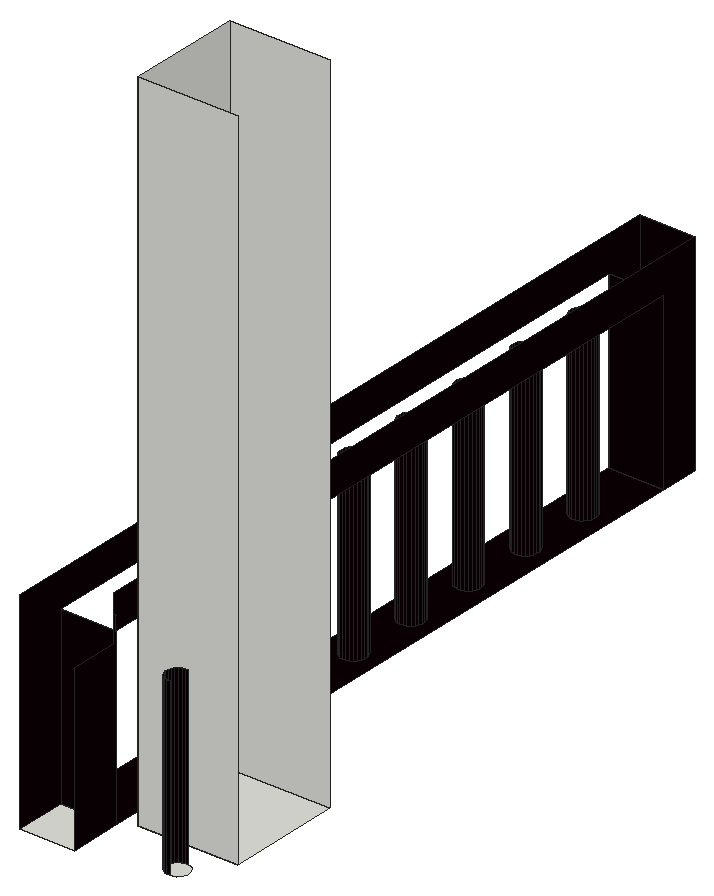
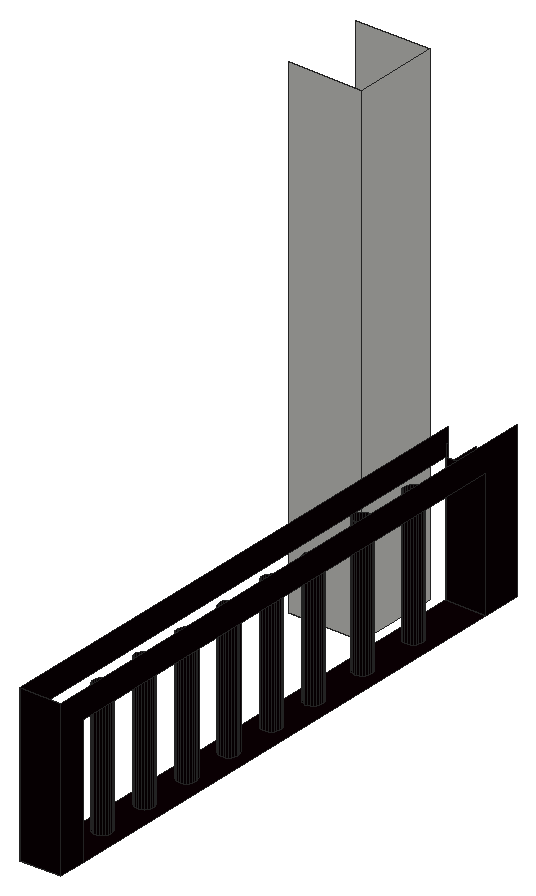
# SketchUp Ruby script. Lengths in inches.
U = 1.inch
M = Sketchup.active_model
def pt(a) = Geom::Point3d.new(a.map { |v| v * U })
def face(e, loops, mat)
  f = e.add_face(loops[0].map { |a| pt(a) })
  loops[1..].each { |l| e.add_face(l.map { |a| pt(a) }).erase! }
  f.material = f.back_material = mat if mat
  f
end
# faces: each face lists its corners as indices into pts; further lists are holes
def faces(e, pts, list, mat = nil) = list.each { |f| face(e, (f[0].is_a?(Array) ? f : [f]).map { |l| l.map { |i| pts[i] } }, mat) }
# xy, xz, yz: faces in a plane at the given z, y or x. An outline is a flat list of corners, or four numbers for a rectangle; further outlines are holes
def ring(l) = l.size == 4 ? [[l[0], l[1]], [l[2], l[1]], [l[2], l[3]], [l[0], l[3]]] : l.each_slice(2).to_a
def flat(e, list, mat, &to3) = list.each { |f| face(e, (f[0].is_a?(Array) ? f : [f]).map { |l| ring(l).map { |u, v| to3.(u, v) } }, mat) }
def xy(e, z, list, mat = nil) = flat(e, list, mat) { |x, y| [x, y, z] }
def xz(e, y, list, mat = nil) = flat(e, list, mat) { |x, z| [x, y, z] }
def yz(e, x, list, mat = nil) = flat(e, list, mat) { |y, z| [x, y, z] }
def lines(e, pts, list) = list.each { |a, b| e.add_line(pt(pts[a]), pt(pts[b])) }
# prism: a flat outline (further loops are holes) pulled along v
def prism(e, loops, v, mat = nil)
  f = face(e, loops, mat); d = Geom::Vector3d.new(v.map { |x| x * U })
  f.pushpull(f.normal.samedirection?(d) ? d.length : -d.length)
end
def box(e, o, s, mat = nil) = prism(e, [[o, [o[0] + s[0], o[1], o[2]], [o[0] + s[0], o[1] + s[1], o[2]], [o[0], o[1] + s[1], o[2]]]], [0, 0, s[2]], mat)
def at(x, y, z, deg = 0) = Geom::Transformation.translation(pt([x, y, z])) * Geom::Transformation.rotation(ORIGIN, Z_AXIS, deg.degrees)
def axes(o, x, y, z) = Geom::Transformation.new([*x, 0, *y, 0, *z, 0, *pt(o).to_a, 1])
def part(name) = M.definitions.add(name)
# library, detail: a bought-in or finely detailed component or shape, given as its bounding box
def library(name, o, s) = part(name).tap { |d| box(d.entities, o, s) }
def detail(e, o, s) = box(e.add_group.entities, o, s)
def put(e, d, t, mat = nil) = e.add_instance(d, t).tap { |i| i.material = mat if mat }
def group(e, t, mat = nil) = e.add_group.tap { |g| g.transformation = t; g.material = mat if mat }.entities
root = M.entities
M.materials.add("[Metal Seamed]").color = [11, 0, 4]
xy(root,148.4375,[[12.3125,62.41,21.75,71.24],[35.91,65.07,35.4,65.08,34.92,65.22,34.48,65.48,34.13,65.84,33.89,66.29,33.76,66.78,33.77,67.28,33.91,67.77,34.17,68.2,34.53,68.55,34.98,68.8,35.47,68.92,35.97,68.91,36.46,68.78,36.89,68.52,37.25,68.15,37.49,67.71,37.61,67.22,37.61,66.71,37.47,66.23,37.21,65.79,36.84,65.44,36.4,65.2],[24.07,73.08,41.19,92.83],[17.07,84.28,16.52,84.4,16.03,84.65,15.62,85.02,15.32,85.49,15.15,86.02,15.125,86.57,15.24,87.12,15.5,87.61,15.87,88.02,16.34,88.32,16.87,88.49,17.42,88.51,17.96,88.4,18.45,88.14,18.87,87.77,19.17,87.3,19.33,86.77,19.36,86.22,19.24,85.68,18.99,85.19,18.62,84.77,18.15,84.47,17.62,84.31],[17.07,99.09,16.52,99.21,16.03,99.46,15.62,99.84,15.32,100.3,15.15,100.83,15.125,101.39,15.24,101.93,15.5,102.42,15.87,102.83,16.34,103.13,16.87,103.3,17.42,103.33,17.96,103.21,18.45,102.96,18.87,102.58,19.17,102.12,19.33,101.59,19.36,101.03,19.24,100.49,18.99,100,18.62,99.59,18.15,99.29,17.62,99.12],
  [17.07,113.4,16.52,113.52,16.03,113.78,15.62,114.15,15.32,114.62,15.15,115.14,15.125,115.7,15.24,116.24,15.5,116.73,15.87,117.14,16.34,117.44,16.87,117.61,17.42,117.64,17.96,117.52,18.45,117.27,18.87,116.89,19.17,116.43,19.33,115.9,19.36,115.35,19.24,114.8,18.99,114.31,18.62,113.9,18.15,113.6,17.62,113.43],[17.07,125.72,16.52,125.83,16.03,126.09,15.62,126.46,15.32,126.93,15.15,127.46,15.125,128.01,15.24,128.55,15.5,129.05,15.87,129.46,16.34,129.76,16.87,129.93,17.42,129.95,17.96,129.83,18.45,129.58,18.87,129.21,19.17,128.74,19.33,128.21,19.36,127.66,19.24,127.12,18.99,126.62,18.62,126.21,18.15,125.91,17.62,125.74],[17.07,138.03,16.52,138.15,16.03,138.4,15.62,138.77,15.32,139.24,15.15,139.77,15.125,140.32,15.24,140.87,15.5,141.36,15.87,141.77,16.34,142.07,16.87,142.24,17.42,142.26,17.96,142.15,18.45,141.89,18.87,141.52,19.17,141.05,19.33,140.52,19.36,139.97,19.24,139.43,18.99,138.94,18.62,138.52,18.15,138.22,17.62,138.06],[17.07,150.34,16.52,150.46,16.03,150.71,15.62,151.09,15.32,151.55,15.15,152.08,15.125,152.64,15.24,153.18,15.5,153.67,15.87,154.08,16.34,154.38,16.87,154.55,17.42,154.58,17.96,154.46,18.45,154.21,18.87,153.83,19.17,153.37,19.33,152.84,19.36,152.28,19.24,151.74,18.99,151.25,18.62,150.84,18.15,150.54,17.62,150.37],[17.07,162.65,16.52,162.77,16.03,163.03,15.62,163.4,15.32,163.87,15.15,164.39,15.125,164.95,15.24,165.49,15.5,165.98,15.87,166.39,16.34,166.69,16.87,166.86,17.42,166.89,17.96,166.77,18.45,166.52,18.87,166.14,19.17,165.68,19.33,165.15,19.36,164.6,19.24,164.05,18.99,163.56,18.62,163.15,18.15,162.85,17.62,162.68],
  [17.07,174.97,16.52,175.08,16.03,175.34,15.62,175.71,15.32,176.18,15.15,176.71,15.125,177.26,15.24,177.8,15.5,178.3,15.87,178.71,16.34,179.01,16.87,179.18,17.42,179.2,17.96,179.08,18.45,178.83,18.87,178.46,19.17,177.99,19.33,177.46,19.36,176.91,19.24,176.37,18.99,175.87,18.62,175.46,18.15,175.16,17.62,174.99],[12.3125,188.85,21.75,195.41]])
xy(root,148.4375,[[[12.3125,71.24,21.75,188.85],[17.07,162.65,16.52,162.77,16.03,163.03,15.62,163.4,15.32,163.87,15.15,164.39,15.125,164.95,15.24,165.49,15.5,165.98,15.87,166.39,16.34,166.69,16.87,166.86,17.42,166.89,17.96,166.77,18.45,166.52,18.87,166.14,19.17,165.68,19.33,165.15,19.36,164.6,19.24,164.05,18.99,163.56,18.62,163.15,18.15,162.85,17.62,162.68],[17.07,150.34,16.52,150.46,16.03,150.71,15.62,151.09,15.32,151.55,15.15,152.08,15.125,152.64,15.24,153.18,15.5,153.67,15.87,154.08,16.34,154.38,16.87,154.55,17.42,154.58,17.96,154.46,18.45,154.21,18.87,153.83,19.17,153.37,19.33,152.84,19.36,152.28,19.24,151.74,18.99,151.25,18.62,150.84,18.15,150.54,17.62,150.37],[17.07,138.03,16.52,138.15,16.03,138.4,15.62,138.77,15.32,139.24,15.15,139.77,15.125,140.32,15.24,140.87,15.5,141.36,15.87,141.77,16.34,142.07,16.87,142.24,17.42,142.26,17.96,142.15,18.45,141.89,18.87,141.52,19.17,141.05,19.33,140.52,19.36,139.97,19.24,139.43,18.99,138.94,18.62,138.52,18.15,138.22,17.62,138.06],[17.07,125.72,16.52,125.83,16.03,126.09,15.62,126.46,15.32,126.93,15.15,127.46,15.125,128.01,15.24,128.55,15.5,129.05,15.87,129.46,16.34,129.76,16.87,129.93,17.42,129.95,17.96,129.83,18.45,129.58,18.87,129.21,19.17,128.74,19.33,128.21,19.36,127.66,19.24,127.12,18.99,126.62,18.62,126.21,18.15,125.91,17.62,125.74],[17.07,113.4,16.52,113.52,16.03,113.78,15.62,114.15,15.32,114.62,15.15,115.14,15.125,115.7,15.24,116.24,15.5,116.73,15.87,117.14,16.34,117.44,16.87,117.61,17.42,117.64,17.96,117.52,18.45,117.27,18.87,116.89,19.17,116.43,19.33,115.9,19.36,115.35,19.24,114.8,18.99,114.31,18.62,113.9,18.15,113.6,17.62,113.43],[17.07,99.09,16.52,99.21,16.03,99.46,15.62,99.84,15.32,100.3,15.15,100.83,15.125,101.39,15.24,101.93,15.5,102.42,15.87,102.83,16.34,103.13,16.87,103.3,17.42,103.33,17.96,103.21,18.45,102.96,18.87,102.58,19.17,102.12,19.33,101.59,19.36,101.03,19.24,100.49,18.99,100,18.62,99.59,18.15,99.29,17.62,99.12],[17.07,84.28,16.52,84.4,16.03,84.65,15.62,85.02,15.32,85.49,15.15,86.02,15.125,86.57,15.24,87.12,15.5,87.61,15.87,88.02,16.34,88.32,16.87,88.49,17.42,88.51,17.96,88.4,18.45,88.14,18.87,87.77,19.17,87.3,19.33,86.77,19.36,86.22,19.24,85.68,18.99,85.19,18.62,84.77,18.15,84.47,17.62,84.31],[17.07,174.97,16.52,175.08,16.03,175.34,15.62,175.71,15.32,176.18,15.15,176.71,15.125,177.26,15.24,177.8,15.5,178.3,15.87,178.71,16.34,179.01,16.87,179.18,17.42,179.2,17.96,179.08,18.45,178.83,18.87,178.46,19.17,177.99,19.33,177.46,19.36,176.91,19.24,176.37,18.99,175.87,18.62,175.46,18.15,175.16,17.62,174.99]]],"[Metal Seamed]")
xz(root,71.24,[[12.3125,148.4375,21.75,178.35]],"[Metal Seamed]")
xz(root,73.08,[[24.07,148.4375,41.19,263.5625]])
xz(root,92.83,[[24.07,148.4375,41.19,263.5625]])
xz(root,188.85,[[12.3125,148.4375,21.75,178.35]],"[Metal Seamed]")
xz(root,195.41,[[12.3125,148.4375,21.75,184.4375]],"[Metal Seamed]")
yz(root,12.3125,[[62.41,148.4375,62.41,184.4375,195.41,184.4375,195.41,148.4375,188.85,148.4375,188.85,178.35,71.24,178.35,71.24,148.4375]],"[Metal Seamed]")
yz(root,21.75,[[62.41,148.4375,71.24,148.4375,71.24,181.04,70.73,181.04,70.73,176.54,62.41,176.54],[188.85,148.4375,195.41,148.4375,195.41,184.4375,70.73,184.4375,70.73,181.04,71.24,181.04,71.24,178.35,188.85,178.35]],"[Metal Seamed]")
yz(root,24.07,[[73.08,148.4375,92.83,263.5625]])
p = [[34.92,65.22,148.4375],[35.4,65.08,148.4375],[35.4,65.08,178.3125],[34.92,65.22,178.3125],[35.91,65.07,148.4375],[35.91,65.07,178.3125],
  [34.48,65.48,148.4375],[34.48,65.48,178.3125],[34.13,65.84,148.4375],[34.13,65.84,178.3125],[33.89,66.29,148.4375],[33.89,66.29,178.3125],
  [33.76,66.78,148.4375],[33.76,66.78,178.3125],[33.77,67.28,148.4375],[33.77,67.28,178.3125],[33.91,67.77,148.4375],[33.91,67.77,178.3125],
  [34.17,68.2,148.4375],[34.17,68.2,178.3125],[34.53,68.55,148.4375],[34.53,68.55,178.3125],[34.98,68.8,148.4375],[34.98,68.8,178.3125],
  [35.47,68.92,148.4375],[35.47,68.92,178.3125],[35.97,68.91,148.4375],[35.97,68.91,178.3125],[16.52,84.4,148.4375],[17.07,84.28,148.4375],
  [17.07,84.28,179.5625],[16.52,84.4,179.5625],[17.62,84.31,148.4375],[17.62,84.31,179.5625],[18.15,84.47,148.4375],[18.15,84.47,179.5625],
  [16.03,84.65,148.4375],[16.03,84.65,179.5625],[18.62,84.77,148.4375],[18.62,84.77,179.5625],[15.62,85.02,148.4375],[15.62,85.02,179.5625],
  [18.99,85.19,148.4375],[18.99,85.19,179.5625],[15.32,85.49,148.4375],[15.32,85.49,179.5625],[19.24,85.68,148.4375],[19.24,85.68,179.5625],
  [15.15,86.02,148.4375],[15.15,86.02,179.5625],[19.36,86.22,148.4375],[19.36,86.22,179.5625],[15.125,86.57,148.4375],[15.125,86.57,179.5625],
  [19.33,86.77,148.4375],[19.33,86.77,179.5625],[15.24,87.12,148.4375],[15.24,87.12,179.5625],[19.17,87.3,148.4375],[19.17,87.3,179.5625],
  [15.5,87.61,148.4375],[15.5,87.61,179.5625],[18.87,87.77,148.4375],[18.87,87.77,179.5625],[15.87,88.02,148.4375],[15.87,88.02,179.5625],
  [18.45,88.14,148.4375],[18.45,88.14,179.5625],[16.34,88.32,148.4375],[16.34,88.32,179.5625],[17.96,88.4,148.4375],[17.96,88.4,179.5625],
  [16.87,88.49,148.4375],[16.87,88.49,179.5625],[17.42,88.51,148.4375],[17.42,88.51,179.5625],[16.52,99.21,148.4375],[17.07,99.09,148.4375],
  [17.07,99.09,180.25],[16.52,99.21,180.25],[17.62,99.12,148.4375],[17.62,99.12,180.25],[18.15,99.29,148.4375],[18.15,99.29,180.25],
  [16.03,99.46,148.4375],[16.03,99.46,180.25],[18.62,99.59,148.4375],[18.62,99.59,180.25],[15.62,99.84,148.4375],[15.62,99.84,180.25],
  [18.99,100,148.4375],[18.99,100,180.25],[15.32,100.3,148.4375],[15.32,100.3,180.25],[19.24,100.49,148.4375],[19.24,100.49,180.25],
  [15.15,100.83,148.4375],[15.15,100.83,180.25],[19.36,101.03,148.4375],[19.36,101.03,180.25],[15.125,101.39,148.4375],[15.125,101.39,180.25],
  [19.33,101.59,148.4375],[19.33,101.59,180.25],[15.24,101.93,148.4375],[15.24,101.93,180.25],[19.17,102.12,148.4375],[19.17,102.12,180.25],
  [15.5,102.42,148.4375],[15.5,102.42,180.25],[18.87,102.58,148.4375],[18.87,102.58,180.25],[15.87,102.83,148.4375],[15.87,102.83,180.25],
  [18.45,102.96,148.4375],[18.45,102.96,180.25],[16.34,103.13,148.4375],[16.34,103.13,180.25],[17.96,103.21,148.4375],[17.96,103.21,180.25],
  [16.87,103.3,148.4375],[16.87,103.3,180.25],[17.42,103.33,148.4375],[17.42,103.33,180.25],[16.52,113.52,148.4375],[17.07,113.4,148.4375],
  [17.07,113.4,178.35],[16.52,113.52,178.35],[17.62,113.43,148.4375],[17.62,113.43,178.35],[18.15,113.6,148.4375],[18.15,113.6,178.35],
  [16.03,113.78,148.4375],[16.03,113.78,178.35],[18.62,113.9,148.4375],[18.62,113.9,178.35],[15.62,114.15,148.4375],[15.62,114.15,178.35],
  [18.99,114.31,148.4375],[18.99,114.31,178.35],[15.32,114.62,148.4375],[15.32,114.62,178.35],[19.24,114.8,148.4375],[19.24,114.8,178.35],
  [15.15,115.14,148.4375],[15.15,115.14,178.35],[19.36,115.35,148.4375],[19.36,115.35,178.35],[15.125,115.7,148.4375],[15.125,115.7,178.35],
  [19.33,115.9,148.4375],[19.33,115.9,178.35],[15.24,116.24,148.4375],[15.24,116.24,178.35],[19.17,116.43,148.4375],[19.17,116.43,178.35],
  [15.5,116.73,148.4375],[15.5,116.73,178.35],[18.87,116.89,148.4375],[18.87,116.89,178.35],[15.87,117.14,148.4375],[15.87,117.14,178.35],
  [18.45,117.27,148.4375],[18.45,117.27,178.35],[16.34,117.44,148.4375],[16.34,117.44,178.35],[17.96,117.52,148.4375],[17.96,117.52,178.35],
  [16.87,117.61,148.4375],[16.87,117.61,178.35],[17.42,117.64,148.4375],[17.42,117.64,178.35],[16.52,125.83,148.4375],[17.07,125.72,148.4375],
  [17.07,125.72,179],[16.52,125.83,179],[17.62,125.74,148.4375],[17.62,125.74,179],[18.15,125.91,148.4375],[18.15,125.91,179],
  [16.03,126.09,148.4375],[16.03,126.09,179],[18.62,126.21,148.4375],[18.62,126.21,179],[15.62,126.46,148.4375],[15.62,126.46,179],
  [18.99,126.62,148.4375],[18.99,126.62,179],[15.32,126.93,148.4375],[15.32,126.93,179],[19.24,127.12,148.4375],[19.24,127.12,179],
  [15.15,127.46,148.4375],[15.15,127.46,179],[19.36,127.66,148.4375],[19.36,127.66,179],[15.125,128.01,148.4375],[15.125,128.01,179],
  [19.33,128.21,148.4375],[19.33,128.21,179],[15.24,128.55,148.4375],[15.24,128.55,179],[19.17,128.74,148.4375],[19.17,128.74,179],
  [15.5,129.05,148.4375],[15.5,129.05,179],[18.87,129.21,148.4375],[18.87,129.21,179],[15.87,129.46,148.4375],[15.87,129.46,179],
  [18.45,129.58,148.4375],[18.45,129.58,179],[16.34,129.76,148.4375],[16.34,129.76,179],[17.96,129.83,148.4375],[17.96,129.83,179],
  [16.87,129.93,148.4375],[16.87,129.93,179],[17.42,129.95,148.4375],[17.42,129.95,179],[16.52,138.15,148.4375],[17.07,138.03,148.4375],
  [17.07,138.03,178.9375],[16.52,138.15,178.9375],[17.62,138.06,148.4375],[17.62,138.06,178.9375],[16.03,138.4,148.4375],[16.03,138.4,178.9375],
  [18.15,138.22,148.4375],[18.15,138.22,178.9375],[18.62,138.52,148.4375],[18.62,138.52,178.9375],[15.62,138.77,148.4375],[15.62,138.77,178.9375],
  [18.99,138.94,148.4375],[18.99,138.94,178.9375],[15.32,139.24,148.4375],[15.32,139.24,178.9375],[19.24,139.43,148.4375],[19.24,139.43,178.9375],
  [15.15,139.77,148.4375],[15.15,139.77,178.9375],[19.36,139.97,148.4375],[19.36,139.97,178.9375],[15.125,140.32,148.4375],[15.125,140.32,178.9375],
  [19.33,140.52,148.4375],[19.33,140.52,178.9375],[15.24,140.87,148.4375],[15.24,140.87,178.9375],[19.17,141.05,148.4375],[19.17,141.05,178.9375],
  [15.5,141.36,148.4375],[15.5,141.36,178.9375],[18.87,141.52,148.4375],[18.87,141.52,178.9375],[15.87,141.77,148.4375],[15.87,141.77,178.9375],
  [18.45,141.89,148.4375],[18.45,141.89,178.9375],[16.34,142.07,148.4375],[16.34,142.07,178.9375],[17.96,142.15,148.4375],[17.96,142.15,178.9375],
  [16.87,142.24,148.4375],[16.87,142.24,178.9375],[17.42,142.26,148.4375],[17.42,142.26,178.9375],[16.52,150.46,148.4375],[17.07,150.34,148.4375],
  [17.07,150.34,178.875],[16.52,150.46,178.875],[17.62,150.37,148.4375],[17.62,150.37,178.875],[18.15,150.54,148.4375],[18.15,150.54,178.875],
  [16.03,150.71,148.4375],[16.03,150.71,178.875],[18.62,150.84,148.4375],[18.62,150.84,178.875],[15.62,151.09,148.4375],[15.62,151.09,178.875],
  [18.99,151.25,148.4375],[18.99,151.25,178.875],[15.32,151.55,148.4375],[15.32,151.55,178.875],[19.24,151.74,148.4375],[19.24,151.74,178.875],
  [15.15,152.08,148.4375],[15.15,152.08,178.875],[19.36,152.28,148.4375],[19.36,152.28,178.875],[15.125,152.64,148.4375],[15.125,152.64,178.875],
  [19.33,152.84,148.4375],[19.33,152.84,178.875],[15.24,153.18,148.4375],[15.24,153.18,178.875],[19.17,153.37,148.4375],[19.17,153.37,178.875],
  [15.5,153.67,148.4375],[15.5,153.67,178.875],[18.87,153.83,148.4375],[18.87,153.83,178.875],[15.87,154.08,148.4375],[15.87,154.08,178.875],
  [18.45,154.21,148.4375],[18.45,154.21,178.875],[16.34,154.38,148.4375],[16.34,154.38,178.875],[17.96,154.46,148.4375],[17.96,154.46,178.875],
  [16.87,154.55,148.4375],[16.87,154.55,178.875],[17.42,154.58,148.4375],[17.42,154.58,178.875],[16.52,162.77,148.4375],[17.07,162.65,148.4375],
  [17.07,162.65,179.0625],[16.52,162.77,179.0625],[17.62,162.68,148.4375],[17.62,162.68,179.0625],[18.15,162.85,148.4375],[18.15,162.85,179.0625],
  [16.03,163.03,148.4375],[16.03,163.03,179.0625],[18.62,163.15,148.4375],[18.62,163.15,179.0625],[15.62,163.4,148.4375],[15.62,163.4,179.0625],
  [18.99,163.56,148.4375],[18.99,163.56,179.0625],[15.32,163.87,148.4375],[15.32,163.87,179.0625],[19.24,164.05,148.4375],[19.24,164.05,179.0625],
  [15.15,164.39,148.4375],[15.15,164.39,179.0625],[19.36,164.6,148.4375],[19.36,164.6,179.0625],[15.125,164.95,148.4375],[15.125,164.95,179.0625],
  [19.33,165.15,148.4375],[19.33,165.15,179.0625],[15.24,165.49,148.4375],[15.24,165.49,179.0625],[19.17,165.68,148.4375],[19.17,165.68,179.0625],
  [15.5,165.98,148.4375],[15.5,165.98,179.0625],[18.87,166.14,148.4375],[18.87,166.14,179.0625],[15.87,166.39,148.4375],[15.87,166.39,179.0625],
  [18.45,166.52,148.4375],[18.45,166.52,179.0625],[16.34,166.69,148.4375],[16.34,166.69,179.0625],[17.96,166.77,148.4375],[17.96,166.77,179.0625],
  [16.87,166.86,148.4375],[16.87,166.86,179.0625],[17.42,166.89,148.4375],[17.42,166.89,179.0625],[16.52,175.08,148.4375],[17.07,174.97,148.4375],
  [17.07,174.97,178.9375],[16.52,175.08,178.9375],[17.62,174.99,148.4375],[17.62,174.99,178.9375],[18.15,175.16,148.4375],[18.15,175.16,178.9375],
  [16.03,175.34,148.4375],[16.03,175.34,178.9375],[18.62,175.46,148.4375],[18.62,175.46,178.9375],[15.62,175.71,148.4375],[15.62,175.71,178.9375],
  [18.99,175.87,148.4375],[18.99,175.87,178.9375],[15.32,176.18,148.4375],[15.32,176.18,178.9375],[19.24,176.37,148.4375],[19.24,176.37,178.9375],
  [15.15,176.71,148.4375],[15.15,176.71,178.9375],[19.36,176.91,148.4375],[19.36,176.91,178.9375],[15.125,177.26,148.4375],[15.125,177.26,178.9375],
  [19.33,177.46,148.4375],[19.33,177.46,178.9375],[15.24,177.8,148.4375],[15.24,177.8,178.9375],[19.17,177.99,148.4375],[19.17,177.99,178.9375],
  [15.5,178.3,148.4375],[15.5,178.3,178.9375],[18.87,178.46,148.4375],[18.87,178.46,178.9375],[15.87,178.71,148.4375],[15.87,178.71,178.9375],
  [18.45,178.83,148.4375],[18.45,178.83,178.9375],[16.34,179.01,148.4375],[16.34,179.01,178.9375],[17.96,179.08,148.4375],[17.96,179.08,178.9375],
  [16.87,179.18,148.4375],[16.87,179.18,178.9375],[17.42,179.2,148.4375],[17.42,179.2,178.9375]]
faces(root,p,[[0,1,2,3],[1,4,5,2],[6,0,3,7],[8,6,7,9],[10,8,9,11],[12,10,11,13],[14,12,13,15],[16,14,15,17],
  [18,16,17,19],[20,18,19,21],[22,20,21,23],[24,22,23,25],[26,24,25,27],[28,29,30,31],[29,32,33,30],[32,34,35,33],
  [36,28,31,37],[34,38,39,35],[40,36,37,41],[38,42,43,39],[44,40,41,45],[42,46,47,43],[48,44,45,49],[46,50,51,47],
  [52,48,49,53],[50,54,55,51],[56,52,53,57],[54,58,59,55],[60,56,57,61],[58,62,63,59],[64,60,61,65],[62,66,67,63],
  [68,64,65,69],[66,70,71,67],[72,68,69,73],[70,74,75,71],[74,72,73,75],[76,77,78,79],[77,80,81,78],[80,82,83,81],
  [84,76,79,85],[82,86,87,83],[88,84,85,89],[86,90,91,87],[92,88,89,93],[90,94,95,91],[96,92,93,97],[94,98,99,95],
  [100,96,97,101],[98,102,103,99],[104,100,101,105],[102,106,107,103],[108,104,105,109],[106,110,111,107],[112,108,109,113],[110,114,115,111],
  [116,112,113,117],[114,118,119,115],[120,116,117,121],[118,122,123,119],[122,120,121,123],[124,125,126,127],[125,128,129,126],[128,130,131,129],
  [132,124,127,133],[130,134,135,131],[136,132,133,137],[134,138,139,135],[140,136,137,141],[138,142,143,139],[144,140,141,145],[142,146,147,143],
  [148,144,145,149],[146,150,151,147],[152,148,149,153],[150,154,155,151],[156,152,153,157],[154,158,159,155],[160,156,157,161],[158,162,163,159],
  [164,160,161,165],[162,166,167,163],[168,164,165,169],[166,170,171,167],[170,168,169,171],[172,173,174,175],[173,176,177,174],[176,178,179,177],
  [180,172,175,181],[178,182,183,179],[184,180,181,185],[182,186,187,183],[188,184,185,189],[186,190,191,187],[192,188,189,193],[190,194,195,191],
  [196,192,193,197],[194,198,199,195],[200,196,197,201],[198,202,203,199],[204,200,201,205],[202,206,207,203],[208,204,205,209],[206,210,211,207],
  [212,208,209,213],[210,214,215,211],[216,212,213,217],[214,218,219,215],[218,216,217,219],[220,221,222,223],[221,224,225,222],[226,220,223,227],
  [224,228,229,225],[228,230,231,229],[232,226,227,233],[230,234,235,231],[236,232,233,237],[234,238,239,235],[240,236,237,241],[238,242,243,239],
  [244,240,241,245],[242,246,247,243],[248,244,245,249],[246,250,251,247],[252,248,249,253],[250,254,255,251],[256,252,253,257],[254,258,259,255],
  [260,256,257,261],[258,262,263,259],[264,260,261,265],[262,266,267,263],[266,264,265,267],[268,269,270,271],[269,272,273,270],[272,274,275,273],
  [276,268,271,277],[274,278,279,275],[280,276,277,281],[278,282,283,279],[284,280,281,285],[282,286,287,283],[288,284,285,289],[286,290,291,287],
  [292,288,289,293],[290,294,295,291],[296,292,293,297],[294,298,299,295],[300,296,297,301],[298,302,303,299],[304,300,301,305],[302,306,307,303],
  [308,304,305,309],[306,310,311,307],[312,308,309,313],[310,314,315,311],[314,312,313,315],[316,317,318,319],[317,320,321,318],[320,322,323,321],
  [324,316,319,325],[322,326,327,323],[328,324,325,329],[326,330,331,327],[332,328,329,333],[330,334,335,331],[336,332,333,337],[334,338,339,335],
  [340,336,337,341],[338,342,343,339],[344,340,341,345],[342,346,347,343],[348,344,345,349],[346,350,351,347],[352,348,349,353],[350,354,355,351],
  [356,352,353,357],[354,358,359,355],[360,356,357,361],[358,362,363,359],[362,360,361,363],[364,365,366,367],[365,368,369,366],[368,370,371,369],
  [372,364,367,373],[370,374,375,371],[376,372,373,377],[374,378,379,375],[380,376,377,381],[378,382,383,379],[384,380,381,385],[382,386,387,383],
  [388,384,385,389],[386,390,391,387],[392,388,389,393],[390,394,395,391],[396,392,393,397],[394,398,399,395],[400,396,397,401],[398,402,403,399],
  [404,400,401,405],[402,406,407,403],[408,404,405,409],[406,410,411,407],[410,408,409,411]],"[Metal Seamed]")
